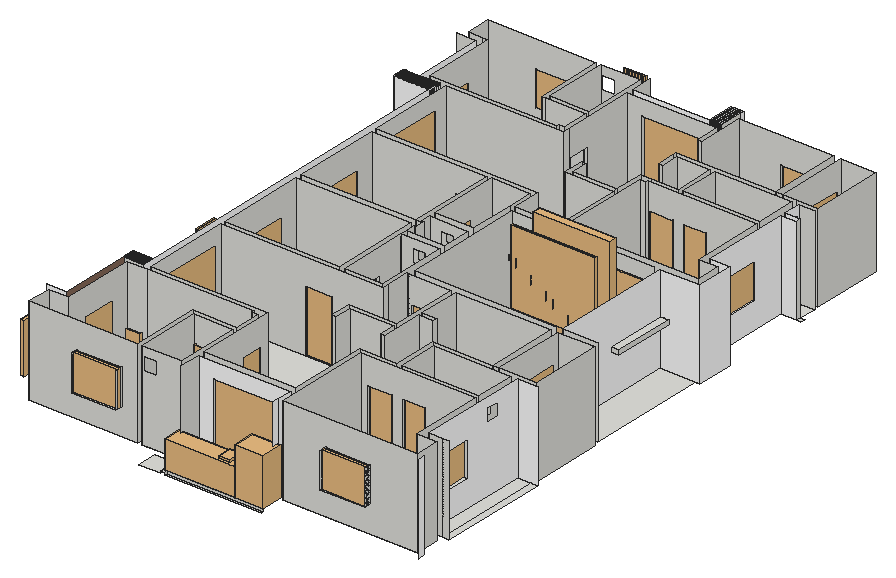
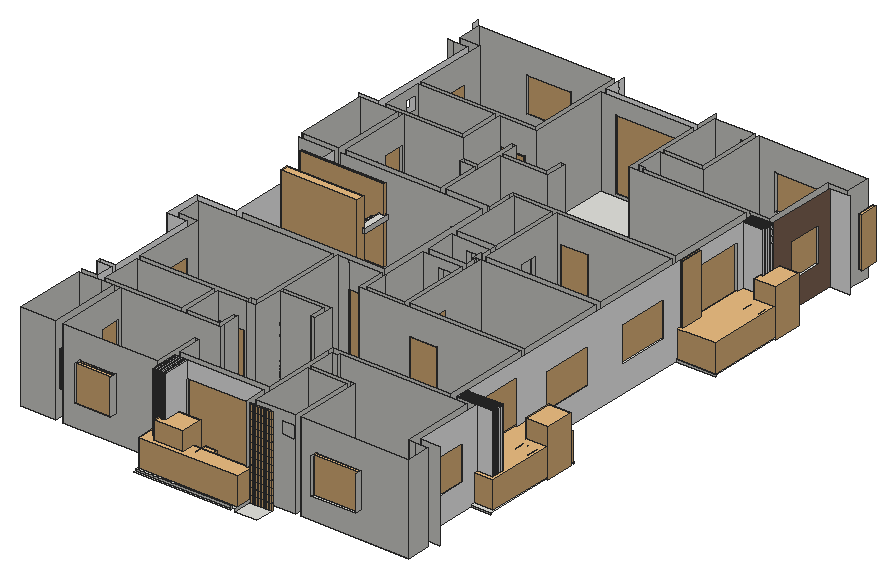
# SketchUp Ruby script. Lengths in inches.
U = 1.inch
M = Sketchup.active_model
def pt(a) = Geom::Point3d.new(a.map { |v| v * U })
def face(e, loops, mat)
  f = e.add_face(loops[0].map { |a| pt(a) })
  loops[1..].each { |l| e.add_face(l.map { |a| pt(a) }).erase! }
  f.material = f.back_material = mat if mat
  f
end
# faces: each face lists its corners as indices into pts; further lists are holes
def faces(e, pts, list, mat = nil) = list.each { |f| face(e, (f[0].is_a?(Array) ? f : [f]).map { |l| l.map { |i| pts[i] } }, mat) }
# xy, xz, yz: faces in a plane at the given z, y or x. An outline is a flat list of corners, or four numbers for a rectangle; further outlines are holes
def ring(l) = l.size == 4 ? [[l[0], l[1]], [l[2], l[1]], [l[2], l[3]], [l[0], l[3]]] : l.each_slice(2).to_a
def flat(e, list, mat, &to3) = list.each { |f| face(e, (f[0].is_a?(Array) ? f : [f]).map { |l| ring(l).map { |u, v| to3.(u, v) } }, mat) }
def xy(e, z, list, mat = nil) = flat(e, list, mat) { |x, y| [x, y, z] }
def xz(e, y, list, mat = nil) = flat(e, list, mat) { |x, z| [x, y, z] }
def yz(e, x, list, mat = nil) = flat(e, list, mat) { |y, z| [x, y, z] }
def lines(e, pts, list) = list.each { |a, b| e.add_line(pt(pts[a]), pt(pts[b])) }
# prism: a flat outline (further loops are holes) pulled along v
def prism(e, loops, v, mat = nil)
  f = face(e, loops, mat); d = Geom::Vector3d.new(v.map { |x| x * U })
  f.pushpull(f.normal.samedirection?(d) ? d.length : -d.length)
end
def box(e, o, s, mat = nil) = prism(e, [[o, [o[0] + s[0], o[1], o[2]], [o[0] + s[0], o[1] + s[1], o[2]], [o[0], o[1] + s[1], o[2]]]], [0, 0, s[2]], mat)
def at(x, y, z, deg = 0) = Geom::Transformation.translation(pt([x, y, z])) * Geom::Transformation.rotation(ORIGIN, Z_AXIS, deg.degrees)
def axes(o, x, y, z) = Geom::Transformation.new([*x, 0, *y, 0, *z, 0, *pt(o).to_a, 1])
def part(name) = M.definitions.add(name)
# library, detail: a bought-in or finely detailed component or shape, given as its bounding box
def library(name, o, s) = part(name).tap { |d| box(d.entities, o, s) }
def detail(e, o, s) = box(e.add_group.entities, o, s)
def put(e, d, t, mat = nil) = e.add_instance(d, t).tap { |i| i.material = mat if mat }
def group(e, t, mat = nil) = e.add_group.tap { |g| g.transformation = t; g.material = mat if mat }.entities
root = M.entities
M.materials.add("T8500 Silicone plaster D1 27.81cm").color = [255, 255, 255]
M.materials.add("Wintan - wpa36452 29.79cm").color = [255, 255, 255]
M.materials.add("Wood Planks C01 100cm").color = [136, 107, 89]
c1 = library("Door 243 053",[-21.6,-2.79,-0.07],[43.2,5.58,82.64])
c2 = library("Group1606\#2",[0.89,0.19,0],[2.1,4.18,2.5])
c3 = library("Potted Plant 13",[-10,-7.28,0],[18.93,15.17,39.22])
c4 = part("Rectangular column")
box(c4.entities,[0,16,0],[27,1,119.8])
box(c4.entities,[0,3.56,0],[27,1,120])
box(c4.entities,[0,1.78,0],[27,1,120])
box(c4.entities,[0,14.22,0],[27,1,119.8])
box(c4.entities,[0,5.33,0],[27,1,120])
box(c4.entities,[0,7.11,0],[27,1,120])
box(c4.entities,[0,10.67,0],[27,1,120.2])
box(c4.entities,[0,12.44,0],[27,1,119.8])
box(c4.entities,[0,0,0],[27,1,120])
xy(c4.entities,0,[[0,8.89,27,9.89]])
xy(c4.entities,120,[[0,8.89,27,9.89]])
xz(c4.entities,8.89,[[0,0,27,120]])
xz(c4.entities,9.89,[[0,0,27,120]])
yz(c4.entities,0,[[8.89,0,9.89,120]],"Wintan - wpa36452 29.79cm")
yz(c4.entities,27,[[8.89,0,9.89,120]])
c5 = part("Stair tread \#1")
box(c5.entities,[0,0,0],[10,39,7])
c6 = part("Stair tread")
box(c6.entities,[0,0,0],[10,39,7])
c7 = part("Group\#9")
box(c7.entities,[100,0,63],[49,84,7])
box(c7.entities,[0,45,0],[20,39,7])
put(c7.entities,c5,at(50,45,28))
put(c7.entities,c5,at(20,45,7))
put(c7.entities,c5,at(90,45,56))
put(c7.entities,c5,at(70,45,42))
put(c7.entities,c5,at(40,45,21))
put(c7.entities,c5,at(60,45,35))
put(c7.entities,c5,at(30,45,14))
put(c7.entities,c5,at(80,45,49))
put(c7.entities,c6,at(90,0,70))
put(c7.entities,c6,at(10,0,126))
put(c7.entities,c6,at(60,0,91))
put(c7.entities,c6,at(30,0,112))
put(c7.entities,c6,at(50,0,98))
put(c7.entities,c6,at(70,0,84))
put(c7.entities,c6,at(80,0,77))
put(c7.entities,c6,at(40,0,105))
put(c7.entities,c6,at(0,0,133))
put(c7.entities,c6,at(20,0,119))
c8 = library("Potted Plant 50-12",[-6.11,-5.26,0],[11.24,10.56,13.41])
c9 = part("Decorative grille insert")
p = [[0.961,0,5],[0.961,0,4.995]]
lines(c9.entities,p,[[0,1]])
detail(c9.entities,[0,0,0],[4.12,1.8,10])
c10 = part("Group\#25")
put(c10.entities,c9,at(0,0,0))
put(c10.entities,c9,at(4.12,0,0))
put(c10.entities,c9,at(8.24,0,0))
put(c10.entities,c9,at(12.36,0,0))
put(c10.entities,c9,at(16.48,0,0))
put(c10.entities,c9,at(20.61,0,0))
put(c10.entities,c9,at(24.73,0,0))
put(c10.entities,c9,at(28.85,0,0))
put(c10.entities,c9,at(0,0,10))
put(c10.entities,c9,at(28.85,0,10))
put(c10.entities,c9,at(24.73,0,10))
put(c10.entities,c9,at(20.61,0,10))
put(c10.entities,c9,at(12.36,0,10))
put(c10.entities,c9,at(16.48,0,10))
put(c10.entities,c9,at(4.12,0,10))
put(c10.entities,c9,at(8.24,0,10))
put(c10.entities,c9,at(0,0,20))
put(c10.entities,c9,at(28.85,0,20))
put(c10.entities,c9,at(24.73,0,20))
put(c10.entities,c9,at(20.61,0,20))
put(c10.entities,c9,at(12.36,0,20))
put(c10.entities,c9,at(16.48,0,20))
put(c10.entities,c9,at(4.12,0,20))
put(c10.entities,c9,at(8.24,0,20))
put(c10.entities,c9,at(0,0,30))
put(c10.entities,c9,at(28.85,0,30))
put(c10.entities,c9,at(24.73,0,30))
put(c10.entities,c9,at(20.61,0,30))
put(c10.entities,c9,at(12.36,0,30))
put(c10.entities,c9,at(16.48,0,30))
put(c10.entities,c9,at(4.12,0,30))
put(c10.entities,c9,at(8.24,0,30))
put(c10.entities,c9,at(0,0,40))
put(c10.entities,c9,at(28.85,0,40))
put(c10.entities,c9,at(24.73,0,40))
put(c10.entities,c9,at(20.61,0,40))
put(c10.entities,c9,at(12.36,0,40))
put(c10.entities,c9,at(16.48,0,40))
put(c10.entities,c9,at(4.12,0,40))
put(c10.entities,c9,at(8.24,0,40))
put(c10.entities,c9,at(0,0,50))
put(c10.entities,c9,at(28.85,0,50))
put(c10.entities,c9,at(24.73,0,50))
put(c10.entities,c9,at(20.61,0,50))
put(c10.entities,c9,at(12.36,0,50))
put(c10.entities,c9,at(16.48,0,50))
put(c10.entities,c9,at(4.12,0,50))
put(c10.entities,c9,at(8.24,0,50))
put(c10.entities,c9,at(0,0,60))
put(c10.entities,c9,at(28.85,0,60))
put(c10.entities,c9,at(24.73,0,60))
put(c10.entities,c9,at(20.61,0,60))
put(c10.entities,c9,at(12.36,0,60))
put(c10.entities,c9,at(16.48,0,60))
put(c10.entities,c9,at(4.12,0,60))
put(c10.entities,c9,at(8.24,0,60))
put(c10.entities,c9,at(0,0,70))
put(c10.entities,c9,at(28.85,0,70))
put(c10.entities,c9,at(24.73,0,70))
put(c10.entities,c9,at(20.61,0,70))
put(c10.entities,c9,at(12.36,0,70))
put(c10.entities,c9,at(16.48,0,70))
put(c10.entities,c9,at(4.12,0,70))
put(c10.entities,c9,at(8.24,0,70))
put(c10.entities,c9,at(0,0,80))
put(c10.entities,c9,at(28.85,0,80))
put(c10.entities,c9,at(24.73,0,80))
put(c10.entities,c9,at(20.61,0,80))
put(c10.entities,c9,at(12.36,0,80))
put(c10.entities,c9,at(16.48,0,80))
put(c10.entities,c9,at(4.12,0,80))
put(c10.entities,c9,at(8.24,0,80))
put(c10.entities,c9,at(0,0,90))
put(c10.entities,c9,at(28.85,0,90))
put(c10.entities,c9,at(24.73,0,90))
put(c10.entities,c9,at(20.61,0,90))
put(c10.entities,c9,at(12.36,0,90))
put(c10.entities,c9,at(16.48,0,90))
put(c10.entities,c9,at(4.12,0,90))
put(c10.entities,c9,at(8.24,0,90))
put(c10.entities,c9,at(0,0,100))
put(c10.entities,c9,at(28.85,0,100))
put(c10.entities,c9,at(24.73,0,100))
put(c10.entities,c9,at(20.61,0,100))
put(c10.entities,c9,at(12.36,0,100))
put(c10.entities,c9,at(16.48,0,100))
put(c10.entities,c9,at(4.12,0,100))
put(c10.entities,c9,at(8.24,0,100))
put(c10.entities,c9,at(0,0,110))
put(c10.entities,c9,at(28.85,0,110))
put(c10.entities,c9,at(24.73,0,110))
put(c10.entities,c9,at(20.61,0,110))
put(c10.entities,c9,at(12.36,0,110))
put(c10.entities,c9,at(16.48,0,110))
put(c10.entities,c9,at(4.12,0,110))
put(c10.entities,c9,at(8.24,0,110))
put(c10.entities,c9,at(0,0,120))
put(c10.entities,c9,at(28.85,0,120))
put(c10.entities,c9,at(24.73,0,120))
put(c10.entities,c9,at(20.61,0,120))
put(c10.entities,c9,at(12.36,0,120))
put(c10.entities,c9,at(16.48,0,120))
put(c10.entities,c9,at(4.12,0,120))
put(c10.entities,c9,at(8.24,0,120))
c11 = library("Potted Plant 02",[-16.98,-19.78,0],[30.04,38.68,37.52])
c12 = library("Window Crafter Sliding",[0,-0.55,0],[84,4.49,96])
c13 = library("Group\#21",[0,0,0],[134.45,23.44,36.98])
c14 = library("Group\#17",[0,0,0],[54.54,138.15,36.98])
c15 = library("Group\#18",[0,0,0],[54.77,134.11,36.98])
c16 = library("Group\#23",[0,0,0],[133.24,24.34,36.98])
c17 = library("Group\#6",[0,0,0],[112.45,3.15,94.27])
c18 = library("Group\#11",[0,0,0],[103.79,11.15,157.27])
c19 = library("Group1671\#2",[0.95,-0.04,0],[2.23,4.74,4.8])
c20 = library("Window Crafter Sliding 6",[0,-0.55,0],[72,4.49,48])
c21 = library("Window Crafter Sliding 2",[0,-0.55,0],[48,4.49,48])
c22 = library("Window Crafter Sliding 5",[0,-0.55,0],[66,4.49,48])
c23 = library("Window Crafter Sliding 3",[0,-0.55,0],[60,4.49,48])
c24 = library("Group\#12",[0,0,0],[113.66,3.15,100.57])
xy(root,252,[[1975.05,473.67,2005.02,500.67],[2011.02,473.67,2141.52,476.67],[2011.02,482.67,2135.52,530.62],[1798.02,509.67,1945.02,509.67,1945.02,602.67,1954.02,602.67,1954.02,596.67,1951.02,596.67,1951.02,509.67,2005.02,509.67,2005.02,596.67,1978.02,596.67,1978.02,602.67,2005.02,602.67,2005.02,605.67,2011.02,605.67,2011.02,635.67,2005.02,635.67,2005.02,638.67,1997.02,638.67,1997.02,641.67,1825.02,641.67,1825.02,542.67,1798.02,542.67],[2141.52,509.67,2324.52,509.67,2324.52,542.67,2297.52,542.67,2297.52,641.67,2228.52,641.67,2228.52,647.67,2198.52,647.67,2198.52,641.67,2184.02,641.67,2184.02,647.67,2152.02,647.67,2152.02,641.67,2141.52,641.67],
  [2011.02,539.67,2135.52,539.67,2135.52,647.67,2186.52,647.67,2186.52,707.67,2267.52,707.67,2267.52,710.67,2276.52,710.67,2276.52,740.67,2267.52,740.67,2267.52,806.67,2138.52,806.67,2138.52,749.67,2158.52,749.67,2158.52,743.67,2138.52,743.67,2138.52,686.67,2132.52,686.67,2132.52,709.17,2072.52,709.17,2072.52,686.67,2066.52,686.67,2066.52,715.17,2132.52,715.17,2132.52,806.67,2117.52,806.67,2117.52,815.67,2078.52,815.67,2078.52,806.67,2072.52,806.67,2072.52,767.67,1852.02,767.67,1852.02,647.67,2011.02,647.67],[2306.52,551.67,2324.52,701.67],[2324.52,551.67,2333.52,701.67],[1795.02,643.17,1816.02,643.17,1816.02,647.67,1843.02,647.67,1843.02,772.17,1795.02,772.17],[2192.52,647.67,2297.52,701.67],
  [2066.52,686.67,2072.52,686.67,2072.52,709.17,2132.52,709.17,2132.52,686.67,2138.52,686.67,2138.52,743.67,2158.52,743.67,2158.52,749.67,2138.52,749.67,2138.52,806.67,2132.52,806.67,2132.52,715.17,2066.52,715.17],[2276.52,707.67,2324.52,806.67],[2324.52,707.67,2327.52,806.67],[1966.02,767.67,2002.02,767.67,2002.02,773.67,2008.02,773.67,2008.02,809.67,2014.02,809.67,2014.02,833.67,2008.02,833.67,2008.02,893.67,1852.02,893.67,1852.02,773.67,1966.02,773.67],[2014.02,773.67,2066.52,869.67],
  [2066.52,806.67,2075.52,806.67,2075.52,980.67,2078.52,980.67,2078.52,989.67,2072.52,989.67,2072.52,1028.67,2002.02,1028.67,2002.02,1022.67,2008.02,1022.67,2008.02,986.67,2014.02,986.67,2014.02,1022.67,2066.52,1022.67,2066.52,926.67,2014.02,926.67,2014.02,962.67,2008.02,962.67,2008.02,902.67,2014.02,902.67,2014.02,917.67,2066.52,917.67,2066.52,878.67,2014.02,878.67,2014.02,869.67,2066.52,869.67],[2075.52,815.67,2207.52,815.67,2207.52,887.67,2267.52,887.67,2267.52,896.67,2138.52,896.67,2138.52,980.67,2117.52,980.67,2117.52,989.67,2078.52,989.67,2078.52,980.67,2075.52,980.67],[2276.52,815.67,2324.52,980.67],[2014.02,878.67,2066.52,878.67,2066.52,917.67,2014.02,917.67,2014.02,905.17,2017.02,905.17,2017.02,891.17,2014.02,891.17],[1852.02,902.67,2008.02,902.67,2008.02,962.67,2014.02,962.67,2014.02,986.67,2008.02,986.67,2008.02,1022.67,2002.02,1022.67,2002.02,1028.67,1966.02,1028.67,1966.02,1022.67,1852.02,1022.67],
  [2014.02,926.67,2066.52,1022.67],[2132.52,980.67,2330.52,980.67,2330.52,1022.67,2321.52,1022.67,2321.52,989.67,2138.52,989.67,2138.52,1118.67,2132.52,1118.67],[2072.52,989.67,2132.52,989.67,2132.52,1081.17,2066.52,1081.17,2066.52,1109.67,2072.52,1109.67,2072.52,1087.17,2132.52,1087.17,2132.52,1127.67,2149.02,1127.67,2149.02,1121.67,2146.52,1121.67,2146.52,1118.67,2138.52,1118.67,2138.52,989.67,2321.52,989.67,2321.52,1022.67,2294.52,1022.67,2294.52,1121.67,2225.52,1121.67,2225.52,1127.67,2195.52,1127.67,2195.52,1121.67,2181.02,1121.67,2181.02,1127.67,2183.52,1127.67,2183.52,1181.67,2138.52,1181.67,2138.52,1157.67,2132.52,1157.67,2132.52,1187.67,2267.52,1187.67,2267.52,1190.67,2276.52,1190.67,2276.52,1220.67,2267.52,1220.67,2267.52,1286.67,2138.52,1286.67,2138.52,1223.67,2132.52,1223.67,2132.52,1256.67,2011.02,1256.67,2011.02,1148.67,1852.02,1148.67,1852.02,1028.67,2072.52,1028.67],[1852.02,1022.67,1966.02,1028.67],[2294.52,1022.67,2330.52,1022.67,2330.52,1031.67,2303.52,1031.67,2303.52,1151.7,2324.52,1151.7,2324.52,1157.7,2303.52,1157.7,2303.52,1181.67,2294.52,1181.67],
  [1795.02,1024.17,1843.02,1148.67],[2189.52,1127.67,2294.52,1181.67],[2324.52,1151.7,2330.52,1157.7],[1825.02,1154.67,1997.02,1154.67,1997.02,1157.67,2005.02,1157.67,2005.02,1160.17,2011.02,1160.17,2011.02,1190.17,2005.02,1190.17,2005.02,1193.67,1978.02,1193.67,1978.02,1199.67,1954.02,1199.67,1954.02,1193.67,1945.02,1193.67,1945.02,1286.67,1798.02,1286.67,1798.02,1253.67,1825.02,1253.67],[2303.52,1157.7,2324.52,1181.67],
  [2276.52,1187.67,2324.52,1286.67],[1951.02,1199.67,2005.02,1286.67],[2011.02,1265.67,2132.52,1286.67],[2011.02,1286.67,2132.52,1286.67,2132.52,1295.67,2135.52,1295.67,2135.52,1313.67,2011.02,1313.67],[1975.05,1295.67,2005.02,1322.67],
  [2011.02,1319.67,2141.52,1322.67]])
xy(root,255,[[2005.02,473.67,2011.02,473.67,2011.02,476.67,2141.52,476.67,2141.52,500.67,2135.52,500.67,2135.52,482.67,2011.02,482.67,2011.02,500.67,2005.02,500.67],[2031.27,530.62,2115.27,539.67],[1789.02,637.17,1816.02,637.17,1816.02,640.17,1792.02,640.17,1792.02,775.17,1843.02,775.17,1843.02,778.17,1789.02,778.17],[1792.02,640.17,1816.02,640.17,1816.02,643.17,1795.02,643.17,1795.02,772.17,1843.02,772.17,1843.02,775.17,1792.02,775.17],[1843.02,673.67,1852.02,757.67],
  [1789.02,1018.17,1843.02,1018.17,1843.02,1024.17,1795.02,1024.17,1795.02,1148.67,1816.02,1148.67,1816.02,1159.17,1789.02,1159.17],[1843.02,1046.67,1852.02,1130.67],[2031.27,1256.67,2115.27,1265.67],[2005.02,1295.67,2011.02,1295.67,2011.02,1313.67,2135.52,1313.67,2135.52,1295.67,2141.52,1295.67,2141.52,1319.67,2011.02,1319.67,2011.02,1322.67,2005.02,1322.67]])
xy(root,288,[[1863.02,500.67,1923.02,509.67],[2199.52,500.67,2259.52,509.67],[1816.02,569.57,1825.02,617.57],[2297.52,569.57,2306.52,617.57],[2267.52,752.67,2276.52,800.67],
  [1843.02,797.67,1852.02,869.67],[1843.02,926.67,1852.02,998.67],[2294.52,1040.67,2303.52,1106.67],[1816.02,1172.67,1825.02,1220.67],[2267.52,1232.67,2276.52,1280.67],
  [1863.02,1286.67,1923.02,1295.67],[2195.52,1286.67,2243.52,1295.67]])
xz(root,476.67,[[2011.02,252,2141.52,255]])
xz(root,482.67,[[2011.02,252,2135.52,255]])
xz(root,509.67,[[[1798.02,252,1945.02,372],[1863.02,288,1923.02,336]],[[1951.02,252,2005.02,372],[1953.02,342,1970.52,360]],[[2141.52,252,2324.52,372],[2199.52,288,2259.52,336]]])
xz(root,530.62,[[[2011.02,252,2135.52,372],[2031.27,255,2115.27,351]]],"T8500 Silicone plaster D1 27.81cm")
xz(root,539.67,[[[2011.02,252,2135.52,372],[2031.27,255,2115.27,351]]])
xz(root,542.67,[[1798.02,252,1825.02,372],[2297.52,252,2324.52,372]])
xz(root,551.67,[[2306.52,252,2324.52,372],[2324.52,252,2333.52,372]])
xz(root,551.67,[[1789.02,252,1816.02,372]],"T8500 Silicone plaster D1 27.81cm")
xz(root,569.57,[[1816.02,288,1825.02,336],[2297.52,288,2306.52,336]])
xz(root,596.67,[[1951.02,252,1954.02,252,1954.02,336,1978.02,336,1978.02,252,2005.02,252,2005.02,372,1951.02,372]])
xz(root,602.67,[[1945.02,252,1945.02,372,2005.02,372,2005.02,252,1978.02,252,1978.02,336,1954.02,336,1954.02,252]])
xz(root,605.67,[[2005.02,252,2011.02,336]])
xz(root,617.57,[[1816.02,288,1825.02,336],[2297.52,288,2306.52,336]])
xz(root,635.67,[[2005.02,252,2011.02,336]])
xz(root,637.17,[[1789.02,252,1816.02,255]])
xz(root,638.67,[[1997.02,252,2005.02,372]])
xz(root,641.67,[[1825.02,252,1852.02,372],[1852.02,252,1997.02,372],[2141.52,252,2152.02,252,2152.02,336,2184.02,336,2184.02,252,2198.52,252,2198.52,336,2228.52,336,2228.52,252,2297.52,252,2297.52,372,2141.52,372]])
xz(root,643.17,[[1795.02,252,1816.02,255]])
xz(root,647.67,[[1816.02,252,1843.02,372],[1852.02,252,2011.02,372],[2135.52,252,2135.52,372,2186.52,372,2186.52,252,2184.02,252,2184.02,336,2152.02,336,2152.02,252],[2192.52,252,2192.52,372,2297.52,372,2297.52,252,2228.52,252,2228.52,336,2198.52,336,2198.52,252]])
xz(root,673.67,[[1843.02,255,1852.02,351]])
xz(root,686.67,[[2066.52,252,2072.52,372],[2132.52,252,2138.52,372]])
xz(root,701.67,[[2192.52,252,2297.52,372]])
xz(root,701.67,[[2306.52,252,2333.52,372]],"T8500 Silicone plaster D1 27.81cm")
xz(root,707.67,[[2186.52,252,2267.52,372],[2267.52,252,2276.52,372],[2276.52,252,2327.52,372]])
xz(root,709.17,[[2072.52,252,2132.52,372]])
xz(root,710.67,[[2267.52,252,2276.52,336]])
xz(root,715.17,[[2066.52,252,2132.52,372]])
xz(root,740.67,[[2267.52,252,2276.52,336]])
xz(root,743.67,[[2138.52,252,2158.52,372]])
xz(root,749.67,[[2138.52,252,2158.52,372]])
xz(root,752.67,[[2267.52,288,2276.52,336]])
xz(root,757.67,[[1843.02,255,1852.02,351]])
xz(root,767.67,[[1852.02,252,1966.02,252,1966.02,336,2002.02,336,2002.02,252,2072.52,252,2072.52,372,1852.02,372]])
xz(root,772.17,[[1795.02,252,1843.02,255]])
xz(root,773.67,[[1852.02,252,1852.02,372,2008.02,372,2008.02,252,2002.02,252,2002.02,336,1966.02,336,1966.02,252],[2014.02,252,2066.52,372]])
xz(root,778.17,[[1789.02,252,1843.02,255]])
xz(root,797.67,[[1843.02,288,1852.02,336]])
xz(root,800.67,[[2267.52,288,2276.52,336]])
xz(root,806.67,[[2072.52,252,2075.52,372],[2075.52,252,2078.52,252,2078.52,336,2117.52,336,2117.52,252,2132.52,252,2132.52,372,2075.52,372],[2138.52,252,2267.52,372],[2276.52,252,2324.52,372],[2324.52,252,2327.52,372]])
xz(root,809.67,[[2008.02,252,2014.02,336]])
xz(root,815.67,[[2075.52,252,2075.52,372,2267.52,372,2267.52,252,2117.52,252,2117.52,336,2078.52,336,2078.52,252],[2276.52,252,2324.52,372]])
xz(root,833.67,[[2008.02,252,2014.02,336]])
xz(root,869.67,[[[2014.02,252,2066.52,372],[2029.77,342,2047.27,360]],[1843.02,288,1852.02,336]])
xz(root,878.67,[[[2014.02,252,2066.52,372],[2029.77,342,2047.27,360]]])
xz(root,891.17,[[2014.02,252,2017.02,372]])
xz(root,893.67,[[1852.02,252,2008.02,372]])
xz(root,902.67,[[1852.02,252,2008.02,372],[2008.02,252,2014.02,372]])
xz(root,905.17,[[2014.02,252,2017.02,372]])
xz(root,917.67,[[[2014.02,252,2066.52,372],[2029.77,342,2047.27,360]]])
xz(root,926.67,[[[2014.02,252,2066.52,372],[2029.77,342,2047.27,360]],[1843.02,288,1852.02,336]])
xz(root,962.67,[[2008.02,252,2014.02,336]])
xz(root,980.67,[[2075.52,252,2078.52,252,2078.52,336,2117.52,336,2117.52,252,2267.52,252,2267.52,372,2075.52,372]])
xz(root,980.67,[[2276.52,252,2330.52,372]],"T8500 Silicone plaster D1 27.81cm")
xz(root,986.67,[[2008.02,252,2014.02,336]])
xz(root,989.67,[[2072.52,252,2072.52,372,2117.52,372,2117.52,336,2078.52,336,2078.52,252],[2117.52,252,2132.52,372],[2138.52,252,2321.52,372]])
xz(root,998.67,[[1843.02,288,1852.02,336]])
xz(root,1018.17,[[1789.02,252,1843.02,255]])
xz(root,1022.67,[[1852.02,252,1966.02,252,1966.02,336,2002.02,336,2002.02,252,2008.02,252,2008.02,372,1852.02,372],[2014.02,252,2066.52,372],[2294.52,252,2321.52,372]])
xz(root,1024.17,[[1795.02,252,1843.02,255]])
xz(root,1028.67,[[1852.02,252,1852.02,372,2072.52,372,2072.52,252,2002.02,252,2002.02,336,1966.02,336,1966.02,252]])
xz(root,1031.67,[[2303.52,252,2330.52,372]],"T8500 Silicone plaster D1 27.81cm")
xz(root,1040.67,[[2294.52,288,2303.52,336]])
xz(root,1046.67,[[1843.02,255,1852.02,351]])
xz(root,1081.17,[[2066.52,252,2132.52,372]])
xz(root,1087.17,[[2072.52,252,2132.52,372]])
xz(root,1106.67,[[2294.52,288,2303.52,336]])
xz(root,1109.67,[[2066.52,252,2072.52,372]])
xz(root,1118.67,[[2138.52,252,2146.52,372]])
xz(root,1121.67,[[2146.52,252,2149.02,252,2149.02,336,2181.02,336,2181.02,252,2195.52,252,2195.52,336,2225.52,336,2225.52,252,2294.52,252,2294.52,372,2146.52,372]])
xz(root,1127.67,[[2132.52,252,2146.52,372],[2146.52,252,2146.52,372,2183.52,372,2183.52,252,2181.02,252,2181.02,336,2149.02,336,2149.02,252],[2189.52,252,2189.52,372,2294.52,372,2294.52,252,2225.52,252,2225.52,336,2195.52,336,2195.52,252]])
xz(root,1130.67,[[1843.02,255,1852.02,351]])
xz(root,1148.67,[[1795.02,252,1816.02,255],[1816.02,252,1843.02,372],[1852.02,252,2011.02,372]])
xz(root,1151.7,[[2303.52,252,2324.52,372]],"T8500 Silicone plaster D1 27.81cm")
xz(root,1154.67,[[1825.02,252,1997.02,372]])
xz(root,1157.67,[[1997.02,252,2005.02,372],[2132.52,252,2138.52,372]])
xz(root,1157.7,[[2303.52,252,2324.52,372]],"T8500 Silicone plaster D1 27.81cm")
xz(root,1159.17,[[1789.02,252,1816.02,255]])
xz(root,1160.17,[[2005.02,252,2011.02,336]])
xz(root,1172.67,[[1816.02,288,1825.02,336]])
xz(root,1181.67,[[2138.52,252,2183.52,372],[2189.52,252,2294.52,372],[2303.52,252,2324.52,372]])
xz(root,1187.67,[[2132.52,252,2267.52,372],[2267.52,252,2276.52,372],[2276.52,252,2294.52,372],[2294.52,252,2324.52,372]])
xz(root,1190.17,[[2005.02,252,2011.02,336]])
xz(root,1190.67,[[2267.52,252,2276.52,336]])
xz(root,1193.67,[[1945.02,252,1951.02,372],[1951.02,252,1954.02,252,1954.02,336,1978.02,336,1978.02,252,2005.02,252,2005.02,372,1951.02,372]])
xz(root,1199.67,[[1951.02,252,1951.02,372,2005.02,372,2005.02,252,1978.02,252,1978.02,336,1954.02,336,1954.02,252]])
xz(root,1220.67,[[2267.52,252,2276.52,336],[1816.02,288,1825.02,336]])
xz(root,1223.67,[[2132.52,252,2138.52,372]])
xz(root,1232.67,[[2267.52,288,2276.52,336]])
xz(root,1244.67,[[1789.02,252,1816.02,372]])
xz(root,1253.67,[[1798.02,252,1816.02,372],[1816.02,252,1825.02,372]])
xz(root,1256.67,[[[2011.02,252,2132.52,372],[2031.27,255,2115.27,351]]])
xz(root,1265.67,[[[2011.02,252,2132.52,372],[2031.27,255,2115.27,351]]],"T8500 Silicone plaster D1 27.81cm")
xz(root,1280.67,[[2267.52,288,2276.52,336]])
xz(root,1286.67,[[[1798.02,252,1945.02,372],[1863.02,288,1923.02,336]],[[1951.02,252,2005.02,372],[1953.02,342,1970.52,360]],[[2138.52,252,2267.52,372],[2195.52,288,2243.52,336]],[2276.52,252,2324.52,372]])
xz(root,1313.67,[[2011.02,252,2135.52,255]])
xz(root,1319.67,[[2011.02,252,2141.52,255]])
yz(root,1795.02,[[643.17,252,772.17,255],[1024.17,252,1148.67,255]])
yz(root,1798.02,[[509.67,252,542.67,372],[1253.67,252,1286.67,372]])
yz(root,1816.02,[[[1159.17,252,1159.17,255,1148.67,255,1148.67,372,1244.67,372,1244.67,252],[1172.67,288,1220.67,336]]],"T8500 Silicone plaster D1 27.81cm")
yz(root,1816.02,[[[551.67,252,551.67,372,647.67,372,647.67,252,643.17,252,643.17,255,637.17,255,637.17,252],[569.57,288,617.57,336]]],"Wood Planks C01 100cm")
yz(root,1825.02,[[[542.67,252,641.67,372],[569.57,288,617.57,336]],[[1154.67,252,1253.67,372],[1172.67,288,1220.67,336]]])
yz(root,1843.02,[[[647.67,252,647.67,372,1148.67,372,1148.67,252,1024.17,252,1024.17,255,1018.17,255,1018.17,252,778.17,252,778.17,255,772.17,255,772.17,252],[1046.67,255,1130.67,351],[673.67,255,757.67,351],[926.67,288,998.67,336],[797.67,288,869.67,336]]],"T8500 Silicone plaster D1 27.81cm")
yz(root,1852.02,[[[647.67,252,767.67,372],[673.67,255,757.67,351]],[[773.67,252,893.67,372],[797.67,288,869.67,336]],[[902.67,252,1022.67,372],[926.67,288,998.67,336]],[[1028.67,252,1148.67,372],[1046.67,255,1130.67,351]]])
yz(root,1863.02,[[500.67,288,509.67,336],[1286.67,288,1295.67,336]])
yz(root,1923.02,[[500.67,288,509.67,336],[1286.67,288,1295.67,336]])
yz(root,1945.02,[[509.67,252,602.67,372],[1193.67,252,1286.67,372]])
yz(root,1951.02,[[509.67,252,596.67,372],[1199.67,252,1286.67,372]])
yz(root,1954.02,[[596.67,252,602.67,336],[1193.67,252,1199.67,336]])
yz(root,1966.02,[[767.67,252,773.67,336],[1022.67,252,1028.67,336]])
yz(root,1978.02,[[596.67,252,602.67,336],[1193.67,252,1199.67,336]])
yz(root,1997.02,[[638.67,252,641.67,372],[1154.67,252,1157.67,372]])
yz(root,2002.02,[[767.67,252,773.67,336],[1022.67,252,1028.67,336]])
yz(root,2005.02,[[473.67,252,500.67,255],[509.67,252,596.67,372],[602.67,252,602.67,372,638.67,372,638.67,252,635.67,252,635.67,336,605.67,336,605.67,252],[1157.67,252,1157.67,372,1193.67,372,1193.67,252,1190.17,252,1190.17,336,1160.17,336,1160.17,252],[1199.67,252,1286.67,372],
  [1295.67,252,1322.67,255]])
yz(root,2008.02,[[773.67,252,773.67,372,893.67,372,893.67,252,833.67,252,833.67,336,809.67,336,809.67,252],[902.67,252,902.67,372,1022.67,372,1022.67,252,986.67,252,986.67,336,962.67,336,962.67,252]])
yz(root,2011.02,[[473.67,252,476.67,255],[482.67,252,500.67,255],[500.67,252,530.62,372],[539.67,252,605.67,252,605.67,336,635.67,336,635.67,252,647.67,252,647.67,372,539.67,372],[1148.67,252,1157.67,372],
  [1157.67,252,1160.17,252,1160.17,336,1190.17,336,1190.17,252,1256.67,252,1256.67,372,1157.67,372],[1265.67,252,1295.67,372],[1295.67,252,1313.67,255],[1319.67,252,1322.67,255]])
yz(root,2014.02,[[773.67,252,809.67,252,809.67,336,833.67,336,833.67,252,869.67,252,869.67,372,773.67,372],[869.67,252,878.67,372],[878.67,252,891.17,372],[902.67,252,905.17,372],[905.17,252,917.67,372],
  [926.67,252,962.67,252,962.67,336,986.67,336,986.67,252,1022.67,252,1022.67,372,926.67,372]])
yz(root,2017.02,[[891.17,252,905.17,372]])
yz(root,2031.27,[[530.62,255,539.67,351],[1256.67,255,1265.67,351]])
yz(root,2066.52,[[686.67,252,715.17,372],[773.67,252,869.67,372],[878.67,252,917.67,372],[926.67,252,989.67,372],[989.67,252,1022.67,372],
  [1081.17,252,1109.67,372]])
yz(root,2072.52,[[686.67,252,709.17,372],[767.67,252,773.67,372],[773.67,252,806.67,372],[989.67,252,1028.67,372],[1087.17,252,1109.67,372]])
yz(root,2075.52,[[815.67,252,980.67,372]])
yz(root,2078.52,[[806.67,252,815.67,336],[980.67,252,989.67,336]])
yz(root,2115.27,[[530.62,255,539.67,351],[1256.67,255,1265.67,351]])
yz(root,2117.52,[[806.67,252,815.67,336],[980.67,252,989.67,336]])
yz(root,2132.52,[[686.67,252,709.17,372],[715.17,252,806.67,372],[989.67,252,1081.17,372],[1081.17,252,1087.17,372],[1087.17,252,1127.67,372],
  [1157.67,252,1181.67,372],[1181.67,252,1187.67,372],[1223.67,252,1256.67,372],[1265.67,252,1295.67,372]])
yz(root,2135.52,[[482.67,252,500.67,255],[539.67,252,647.67,372],[1295.67,252,1313.67,255]])
yz(root,2135.52,[[500.67,252,509.67,372],[509.67,252,530.62,372]],"T8500 Silicone plaster D1 27.81cm")
yz(root,2138.52,[[686.67,252,743.67,372],[749.67,252,806.67,372],[989.67,252,1118.67,372],[1157.67,252,1181.67,372],[1223.67,252,1286.67,372]])
yz(root,2141.52,[[509.67,252,641.67,372]])
yz(root,2146.52,[[1118.67,252,1121.67,372]])
yz(root,2149.02,[[1121.67,252,1127.67,336]])
yz(root,2152.02,[[641.67,252,647.67,336]])
yz(root,2158.52,[[743.67,252,749.67,372]])
yz(root,2181.02,[[1121.67,252,1127.67,336]])
yz(root,2183.52,[[1127.67,252,1181.67,372]])
yz(root,2184.02,[[641.67,252,647.67,336]])
yz(root,2186.52,[[647.67,252,707.67,372]])
yz(root,2189.52,[[1127.67,252,1181.67,372]])
yz(root,2192.52,[[647.67,252,701.67,372]])
yz(root,2195.52,[[1121.67,252,1127.67,336],[1286.67,288,1295.67,336]])
yz(root,2198.52,[[641.67,252,647.67,336]])
yz(root,2199.52,[[500.67,288,509.67,336]])
yz(root,2225.52,[[1121.67,252,1127.67,336]])
yz(root,2228.52,[[641.67,252,647.67,336]])
yz(root,2243.52,[[1286.67,288,1295.67,336]])
yz(root,2259.52,[[500.67,288,509.67,336]])
yz(root,2267.52,[[[707.67,252,707.67,372,806.67,372,806.67,252,740.67,252,740.67,336,710.67,336,710.67,252],[752.67,288,800.67,336]],[[1187.67,252,1187.67,372,1286.67,372,1286.67,252,1220.67,252,1220.67,336,1190.67,336,1190.67,252],[1232.67,288,1280.67,336]]])
yz(root,2276.52,[[[707.67,252,710.67,252,710.67,336,740.67,336,740.67,252,806.67,252,806.67,372,707.67,372],[752.67,288,800.67,336]],[[1187.67,252,1190.67,252,1190.67,336,1220.67,336,1220.67,252,1286.67,252,1286.67,372,1187.67,372],[1232.67,288,1280.67,336]]])
yz(root,2276.52,[[815.67,252,980.67,372]],"T8500 Silicone plaster D1 27.81cm")
yz(root,2294.52,[[[1022.67,252,1121.67,372],[1040.67,288,1106.67,336]],[[1127.67,252,1181.67,372],[1162.17,342,1179.67,360]]])
yz(root,2297.52,[[[542.67,252,641.67,372],[569.57,288,617.57,336]],[[647.67,252,701.67,372],[649.73,342,667.23,360]]])
yz(root,2303.52,[[[1031.67,252,1151.7,372],[1040.67,288,1106.67,336]],[[1157.7,252,1181.67,372],[1162.17,342,1179.67,360]]],"T8500 Silicone plaster D1 27.81cm")
yz(root,2306.52,[[[551.67,252,701.67,372],[569.57,288,617.57,336],[649.73,342,667.23,360]]],"T8500 Silicone plaster D1 27.81cm")
yz(root,2321.52,[[989.67,252,1022.67,372]])
yz(root,2324.52,[[509.67,252,542.67,372],[1151.7,252,1157.7,372],[1187.67,252,1286.67,372]])
yz(root,2327.52,[[707.67,252,806.67,372]])
yz(root,2330.52,[[980.67,252,1031.67,372]],"T8500 Silicone plaster D1 27.81cm")
yz(root,2333.52,[[500.67,252,509.67,372]],"T8500 Silicone plaster D1 27.81cm")
p = [[2138.52,896.67,252],[2138.52,980.67,252],[2267.52,980.67,252],[2267.52,896.67,252],[2297.52,641.67,252],[2297.52,647.67,252],
  [2143.35,500.67,252],[2141.52,500.67,252]]
lines(root,p,[[0,1],[1,2],[2,3],[3,0],[4,5],[6,7]])
put(root,c1,axes([2213.52,646.74,251.43],[0.69441,0,0],[0,0.74,0],[0,0,1.01843]))
put(root,c1,axes([2168.02,646.74,251.43],[0.7407,0,0],[0,0.74,0],[0,0,1.01843]))
put(root,c1,axes([2273.94,1205.63,251.86],[0,-0.69441,0],[0.74,0,0],[0,0,1.01843]))
put(root,c1,axes([1966.02,1196.98,251.91],[0.55552,0,0],[0,0.74,0],[0,0,1.01843]))
put(root,c1,axes([1984.02,771.84,251.91],[0.83329,0,0],[0,0.74,0],[0,0,1.01843]))
put(root,c1,axes([1984.02,1027.84,251.91],[0.83329,0,0],[0,0.74,0],[0,0,1.01843]))
put(root,c2,axes([1841.02,784.99,246.42],[0,-14.41,0],[0,0,28.70953],[-1,0,0]))
put(root,c1,axes([1965.99,597.61,252],[-0.55696,0,0],[0,-1.07698,0],[0,0,1.01843]))
put(root,c3,at(2066.61,1296.4375,252,90))
put(root,c3,at(1804.9375,1080.65,252))
put(root,c3,at(1804.9375,694.48,252))
put(root,c4,axes([2132.52,1265.67,252],[0,1.33704,0],[-1,0,0],[0,0,0.99834]),"Wintan - wpa36452 29.79cm")
put(root,c7,axes([2138.52,896.67,252],[1,0,0],[0,1,0],[0,0,0.9]))
put(root,c8,axes([2023.09,1300,252],[0,1.65,0],[-1,0,0],[0,0,2]))
put(root,c1,axes([2097.77,811.09,252.07],[0.9143,0,0],[0,0.74,0],[0,0,1.01843]))
put(root,c1,axes([2011.02,974.68,252.07],[0,-0.55585,0],[1.07698,0,0],[0,0,1.01843]))
put(root,c1,axes([2210.52,1123.74,252.07],[0.69441,0,0],[0,0.74,0],[0,0,1.01843]))
put(root,c1,axes([2165.02,1123.74,252.07],[0.7407,0,0],[0,0.74,0],[0,0,1.01843]))
put(root,c1,axes([2097.77,985.74,252.07],[0.9143,0,0],[0,0.74,0],[0,0,1.01843]))
put(root,c4,at(1816.02,647.67,252),"Wintan - wpa36452 29.79cm")
put(root,c1,axes([2006.02,620.3,252.07],[0,-0.71149,0],[1.07698,0,0],[0,0,1.01843]))
put(root,c10,axes([1975.05,1295.67,252],[0.90915,0,0],[0,1,0],[0,0,0.92482]))
put(root,c1,axes([2274.59,725.67,252.07],[0,-0.69441,0],[0.74,0,0],[0,0,1.01843]))
put(root,c11,axes([2104.14,1297.51,252],[0,1,0],[-1,0,0],[0,0,1.71]))
put(root,c8,axes([1808.5,738,252],[1.65,0,0],[0,1,0],[0,0,2]))
put(root,c8,axes([1808.5,1124.17,252],[1.65,0,0],[0,1,0],[0,0,2]))
put(root,c11,axes([1806.01,1043.12,252],[1,0,0],[0,1,0],[0,0,1.71]))
put(root,c11,axes([1806.01,656.95,252],[1,0,0],[0,1,0],[0,0,1.71]))
put(root,c4,axes([1795.02,1131.67,253.46],[1.77778,0,0],[0,1,0],[0,0,0.98781]),"Wintan - wpa36452 29.79cm")
put(root,c3,at(2084.22,492.59,255,90))
put(root,c8,axes([2040.7,496.15,255],[0,1.65,0],[-1,0,0],[0,0,2]))
put(root,c11,axes([2121.74,493.66,255],[0,1,0],[-1,0,0],[0,0,1.71]))
put(root,c12,at(2031.27,533.26,255))
put(root,c12,at(1849.22,1046.67,255,90))
put(root,c12,at(2031.27,1259.48,255))
put(root,c12,at(1851.46,673.67,255,90))
put(root,c13,at(2005.77,1293.7,255))
put(root,c14,at(1790.45,638.6,255))
put(root,c15,at(1790.22,1019.37,255))
put(root,c16,at(2006.65,478.3,255))
put(root,c17,at(2152.15,978.1,258.3))
put(root,c18,at(2141.95,933.1,258.3))
put(root,c19,axes([1789.02,546.03,277.28],[0,-10.69,0],[0,0,14.25642],[-1,0,0]))
put(root,c20,at(1844.98,998.67,288,-90))
put(root,c21,at(2270.52,1280.67,288,-90))
put(root,c21,at(1818.83,1220.67,288,-90))
put(root,c20,at(1847.52,869.67,288,-90))
put(root,c22,at(2300.72,1040.67,288,90))
put(root,c23,at(2199.52,503.48,288))
put(root,c21,at(1820.52,617.57,288,-90))
put(root,c23,at(1863.02,503.48,288))
put(root,c21,at(2270.52,800.67,288,-90))
put(root,c23,at(1863.02,1287.79,288))
put(root,c21,at(2297.52,617.57,288,-90))
put(root,c21,at(2243.52,1293.71,288,180))
put(root,c24,at(2141.95,896.1,315))
